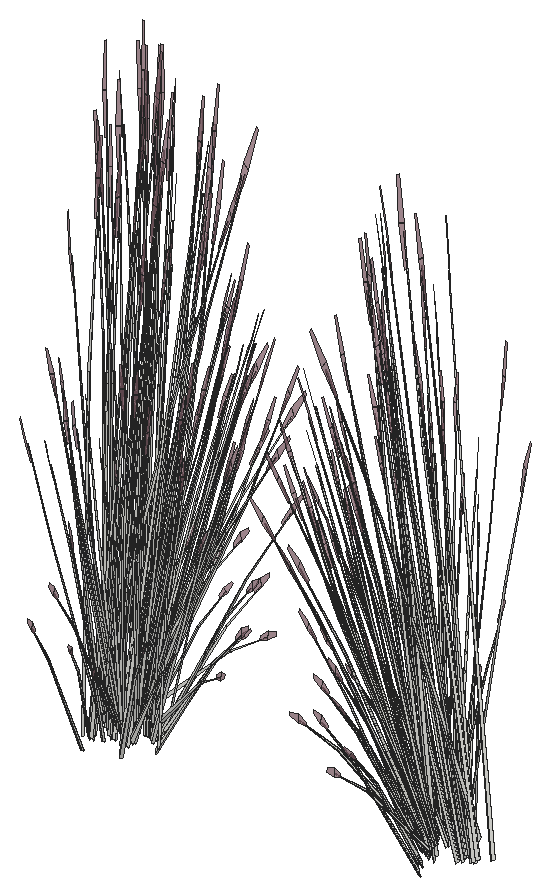
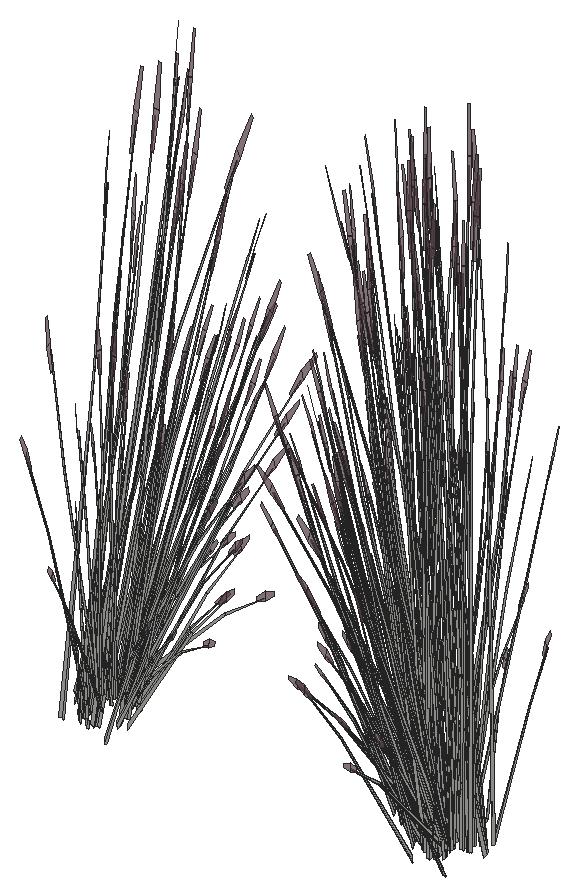
# SketchUp Ruby script. Lengths in inches.
U = 1.inch
M = Sketchup.active_model
def pt(a) = Geom::Point3d.new(a.map { |v| v * U })
def face(e, loops, mat)
  f = e.add_face(loops[0].map { |a| pt(a) })
  loops[1..].each { |l| e.add_face(l.map { |a| pt(a) }).erase! }
  f.material = f.back_material = mat if mat
  f
end
# faces: each face lists its corners as indices into pts; further lists are holes
def faces(e, pts, list, mat = nil) = list.each { |f| face(e, (f[0].is_a?(Array) ? f : [f]).map { |l| l.map { |i| pts[i] } }, mat) }
# xy, xz, yz: faces in a plane at the given z, y or x. An outline is a flat list of corners, or four numbers for a rectangle; further outlines are holes
def ring(l) = l.size == 4 ? [[l[0], l[1]], [l[2], l[1]], [l[2], l[3]], [l[0], l[3]]] : l.each_slice(2).to_a
def flat(e, list, mat, &to3) = list.each { |f| face(e, (f[0].is_a?(Array) ? f : [f]).map { |l| ring(l).map { |u, v| to3.(u, v) } }, mat) }
def xy(e, z, list, mat = nil) = flat(e, list, mat) { |x, y| [x, y, z] }
def xz(e, y, list, mat = nil) = flat(e, list, mat) { |x, z| [x, y, z] }
def yz(e, x, list, mat = nil) = flat(e, list, mat) { |y, z| [x, y, z] }
def lines(e, pts, list) = list.each { |a, b| e.add_line(pt(pts[a]), pt(pts[b])) }
# prism: a flat outline (further loops are holes) pulled along v
def prism(e, loops, v, mat = nil)
  f = face(e, loops, mat); d = Geom::Vector3d.new(v.map { |x| x * U })
  f.pushpull(f.normal.samedirection?(d) ? d.length : -d.length)
end
def box(e, o, s, mat = nil) = prism(e, [[o, [o[0] + s[0], o[1], o[2]], [o[0] + s[0], o[1] + s[1], o[2]], [o[0], o[1] + s[1], o[2]]]], [0, 0, s[2]], mat)
def at(x, y, z, deg = 0) = Geom::Transformation.translation(pt([x, y, z])) * Geom::Transformation.rotation(ORIGIN, Z_AXIS, deg.degrees)
def axes(o, x, y, z) = Geom::Transformation.new([*x, 0, *y, 0, *z, 0, *pt(o).to_a, 1])
def part(name) = M.definitions.add(name)
# library, detail: a bought-in or finely detailed component or shape, given as its bounding box
def library(name, o, s) = part(name).tap { |d| box(d.entities, o, s) }
def detail(e, o, s) = box(e.add_group.entities, o, s)
def put(e, d, t, mat = nil) = e.add_instance(d, t).tap { |i| i.material = mat if mat }
def group(e, t, mat = nil) = e.add_group.tap { |g| g.transformation = t; g.material = mat if mat }.entities
root = M.entities
M.materials.add("LightPink_Translucent").color = [144, 107, 117]
M.materials["LightPink_Translucent"].alpha = 0.75
c1 = part("blade")
p = [[2.15,0.21,22],[0,0.17,0],[0.09,0.45,0],[2.18,0.31,22],[2.29,0.31,22],[0.38,0.45,0],
  [2.48,0.24,33],[2.49,0.24,33],[2.48,0.22,33]]
faces(c1.entities,p,[[0,1,2,3],[4,5,2,3],[6,3,4,7],[8,0,3,6]])
c2 = part("seeds")
p = [[0.3,-0.1,1.38],[-0.01,-0.03,1.59],[-0.01,-0.03,0.03],[0.14,-0.07,-0.07],[0.29,-0.03,3],[0.15,0.01,3.11]]
faces(c2.entities,p,[[0,1,2,3],[1,0,4,5]],"LightPink_Translucent")
c3 = part("blade with seeds")
put(c3.entities,c1,at(0,0,0))
put(c3.entities,c2,axes([2.4,0.25,30.99],[1.5799,-0.05474,1.17369],[-0.12525,1.92788,0.29478],[-0.07173,-0.02425,1.56792]))
put(root,c3,axes([149.6,15.09,-3.67],[0.95122,0.19861,0.30756],[-0.23797,0.7099,-0.36492],[-0.15744,0.08885,1.64885]))
put(root,c3,axes([148.22,9.64,-4.51],[-0.12744,0.02202,1.76342],[-0.70477,-0.24781,-0.26939],[0.01183,-0.2067,0.30037]))
put(root,c3,axes([150.01,15.05,-3.52],[0.7111,-0.30552,0.49651],[0.42504,0.54784,0],[-0.16196,0.06958,1.57504]))
put(root,c3,axes([148.91,10.32,-1.47],[0.22906,-0.4699,-0.35414],[0.66828,0.13705,0.4572],[-0.06128,-0.18919,0.87481]))
put(root,c3,axes([147.79,12.86,-3.64],[0.33034,0.68327,0.45755],[-0.94388,0.2376,0.17955],[0.01154,-0.12555,1.58856]))
put(root,c3,axes([147.64,12.77,-3.79],[0.36864,-0.55059,-0.44739],[0.76598,0.26498,0.21531],[0,-0.12692,1.43643]))
put(root,c3,axes([148.58,14.55,-3.8],[-0.24791,-0.5268,0],[0.70791,-0.18448,0],[0,0,1.54371]))
put(root,c3,axes([147.68,15.66,-4.51],[0.12297,-0.03325,1.76342],[0.73967,0.18301,-0.26939],[0.02163,0.20626,0.30037]))
put(root,c3,axes([147.85,15.84,-1.47],[-0.22906,0.4699,-0.35414],[-0.66828,-0.13705,0.4572],[0.06128,0.18919,0.87481]))
put(root,c3,axes([149.58,13.51,-3.79],[-0.36864,0.55059,-0.44739],[-0.76598,-0.26498,0.21531],[0,0.12692,1.43643]))
put(root,c3,axes([149.19,10.39,-1.27],[0.55987,-0.20767,0.0643],[0.27403,0.37869,0.50621],[-0.05407,-0.16693,0.77189]))
put(root,c3,axes([147.37,16.68,-1.28],[0.09631,0.0984,1.74944],[0.77725,0.03866,-0.27667],[0.07816,0.217,0.14031]))
put(root,c3,axes([151.04,13.17,-3.53],[-0.59697,-0.44509,0.17642],[0.60159,-0.4317,0.35086],[-0.06593,0.0909,1.60407]))
put(root,c3,axes([148.98,12.92,-3.79],[0,-0.70701,0],[0.95008,0,0],[0,0,1.79456]))
put(root,c3,axes([148.99,10.43,-1.27],[0.74868,0.15974,0.48003],[-0.25601,0.52518,0.3958],[-0.04499,-0.20653,0.9933]))
put(root,c3,axes([148.1,13.04,-3.57],[0.8561,0.29616,0.24065],[-0.41201,0.61537,0.50002],[0,-0.14185,1.60543]))
put(root,c3,axes([149.46,13.2,-3.71],[0,0.70667,-0.05637],[-0.95008,0,0],[0,0.02221,1.79368]))
put(root,c3,axes([147.82,12.63,-3.28],[-0.82508,0.03772,0.44739],[-0.07462,-0.62614,-0.21531],[0.14771,-0.06346,1.43643]))
put(root,c3,axes([147.77,15.35,-0.95],[0.22906,-0.4699,0.35414],[0.66828,0.13705,-0.4572],[0.06128,0.18919,0.87481]))
put(root,c3,axes([147.43,11.56,-3.53],[-0.21949,0.60727,0.17642],[-0.8032,-0.17185,0.35086],[0.13875,-0.00296,1.60407]))
put(root,c3,axes([149,14.57,-3.71],[0.33034,0.70197,-0.06012],[-0.94388,0.24598,0],[0.01154,0.02451,1.72173]))
put(root,c3,axes([147.04,10.81,-3.625],[-0.47504,-0.61229,0],[0.79476,-0.34146,-0.51607],[0.18101,-0.07777,1.63711]))
put(root,c3,axes([147.91,15.42,-1.02],[0.36264,0.49684,-0.71045],[-0.74649,0.27689,0.08574],[0.0848,0.24006,1.00501]))
put(root,c3,axes([151.73,13.64,-3.8],[-0.94962,-0.00489,-0.04976],[0,-0.68292,0.49943],[-0.02984,0.15546,1.58352]))
put(root,c3,axes([149.86,11.59,-3.53],[-0.81646,0.16218,0.17642],[-0.20161,-0.60355,0.35086],[0.07282,0.08794,1.60407]))
put(root,c3,axes([149.03,9.33,-3.23],[0.09747,0.35631,1.1486],[-0.54071,-0.19735,0.84392],[0.05818,-0.18244,0.25299]))
put(root,c3,axes([148.67,17.03,-0.35],[0.52505,-0.35054,-0.06488],[0.48109,0.38392,-0.29416],[0.03387,0.10878,0.97024]))
put(root,c3,axes([148.53,12.47,-3.64],[-0.62999,0.55453,0.45755],[-0.74845,-0.4895,0.17955],[0.15188,-0.05534,1.58856]))
put(root,c3,axes([149.6,13.34,-3.79],[0.53038,0.39469,0],[-0.53038,0.39469,0],[0,0,1.69266]))
put(root,c3,axes([149.6,12.88,-3.28],[0.36864,-0.55059,0.44739],[0.76598,0.26498,-0.21531],[0,0.12692,1.43643]))
put(root,c3,axes([149.28,14.8,-3.8],[0.76598,0.27433,0],[-0.36864,0.57001,0],[0,0,1.74954]))
put(root,c3,axes([148.1875,15.52,-1.32],[0.7469,0.15318,-0.51099],[-0.25601,0.52518,-0.3958],[0.06849,0.21144,0.97773]))
put(root,c3,axes([147.55,15.55,-0.97],[0.74352,-0.28449,-0.1216],[0.36538,0.50492,-0.67495],[0.0981,0.21277,1.02557]))
put(root,c3,axes([149.35,12.75,-3.62],[-0.96033,-0.12874,0.49198],[0.19544,-0.7271,0.19306],[0.14034,0.07021,1.70813]))
put(root,c3,axes([151.35,9.91,-1.29],[-0.07716,0.04667,1.77383],[-0.75601,-0.15746,-0.16761],[-0.02737,-0.20368,0.31391]))
put(root,c3,axes([150.75,11.26,-0.97],[-0.83505,-0.03027,-0.1216],[0.02282,-0.57322,-0.67495],[0.05801,-0.22077,1.02557]))
put(root,c3,axes([151.53,13.74,-3.97],[-0.53038,0.38124,-0.30978],[-0.53038,-0.38124,0.30978],[0,0.1228,1.38974]))
put(root,c3,axes([150.02,13.67,-3.91],[0.2786,0.55945,-0.69212],[-0.80253,0.20149,-0.18165],[0.03079,0.18945,1.52773]))
put(root,c3,axes([149.625,13.07,-3.79],[0.85008,0,0],[0,0.63259,0],[0,0,1.78407]))
put(root,c3,axes([150.43,11.35,-0.95],[-0.5141,0.32171,0.35414],[-0.48666,-0.36734,-0.4572],[0.07405,-0.18664,0.87481]))
put(root,c3,axes([148.81,12.375,-3.28],[-0.45644,-0.51287,0.44739],[0.69137,-0.36116,-0.21531],[0.14771,0.06346,1.43643]))
put(root,c3,axes([147.98,12.5,-3.33],[-0.08854,-0.69723,-0.29095],[0.92215,-0.04216,-0.50002],[0.16238,-0.09287,1.59708]))
put(root,c3,axes([149.92,13.01,-3.38],[0.70791,-0.1782,0.1448],[0.24791,0.50885,-0.41347],[0,0.11199,1.26744]))
put(root,c3,axes([150.18,11.04,-1.32],[-0.54391,-0.41056,-0.51099],[0.57458,-0.35956,-0.3958],[0.08276,-0.2086,0.97773]))
put(root,c3,axes([149.68,13.05,-3.33],[0.85568,0.29155,-0.29095],[-0.41201,0.61537,-0.50002],[0.02689,0.15109,1.59708]))
put(root,c3,axes([147.85,10.95,-3.97],[0.70886,0.15119,-0.30978],[-0.17848,0.53243,0.30978],[0.1429,-0.0614,1.38974]))
put(root,c3,axes([149.83,10.3125,-3.41],[-0.21597,0.12368,1.43002],[-0.64681,-0.21647,-0.30754],[0.1199,-0.26922,0.61141]))
put(root,c3,axes([151.53,13.19,-3.52],[0,-0.61104,0.49651],[0.85008,0,0],[0,0.13917,1.57504]))
put(root,c3,axes([151.9,13.76,-3.98],[0,0.61104,-0.49651],[-0.85008,0,0],[0,0.13917,1.57504]))
put(root,c3,axes([149.63,15.61,-1.27],[-0.75571,0.14023,0.48003],[-0.13115,-0.55007,0.3958],[0.17773,0.16212,0.9933]))
put(root,c3,axes([147.6875,10.71,-3.98],[0.7111,-0.30552,-0.49651],[0.42504,0.54784,0],[0.16196,-0.06958,1.57504]))
put(root,c3,axes([149.48,15.72,-1.27],[-0.34533,0.38816,0.0643],[-0.49176,-0.22599,0.50621],[0.15898,0.12445,0.77189]))
put(root,c3,axes([148.61,14.4375,-2.125],[-0.17368,-0.19618,1.71376],[0.80256,-0.16516,0.13857],[0.18139,0.30799,0.73262]))
put(root,c3,axes([149.11,12.23,-3.38],[0.14658,-0.54532,0.1448],[0.71613,0.09466,-0.41347],[0.13033,0.05599,1.26744]))
put(root,c3,axes([150.13,11.28,-3.52],[-0.7111,-0.30552,0.49651],[0.42504,-0.54784,0],[0.16196,0.06958,1.57504]))
put(root,c3,axes([150.35,11.23,-1.02],[0.01977,-0.56521,-0.71045],[0.83252,0.03796,0.08574],[0.08786,-0.23945,1.00501]))
put(root,c3,axes([149.51,14.47,-3.82],[0.79769,-0.20732,-0.19198],[0.2803,0.59721,0.00008],[0.08805,-0.02292,1.73897]))
put(root,c3,axes([149.375,15.27,-0.95],[-0.11735,-0.49217,0.35414],[0.67083,-0.12996,-0.4572],[0.18018,0.14104,0.87481]))
put(root,c3,axes([149.53,12.7,-3.79],[0.45644,0.51287,-0.44739],[-0.69137,0.36116,0.21531],[0.14771,0.06346,1.43643]))
put(root,c3,axes([149.83,12.44,-1.53],[-0.65655,-0.31748,1.38283],[0.69326,-0.49431,0.59665],[0.21183,0.29789,1.33663]))
put(root,c3,axes([150.69,10.89,-1.47],[0.5141,-0.32171,-0.35414],[0.48666,0.36734,0.4572],[0.07405,-0.18664,0.87481]))
put(root,c3,axes([148.72,15.96,-1.29],[0.00225,-0.07398,1.77383],[0.65113,-0.32638,-0.16761],[0.22617,0.1165,0.31391]))
put(root,c3,axes([150.89,11.05,-1.27],[0.62439,0.02847,0.0643],[-0.01712,0.42991,0.50621],[0.06534,-0.16468,0.77189]))
put(root,c3,axes([150.82,15.02,-3.23],[-0.4278,-0.1757,1.1486],[0.5524,-0.17852,0.84392],[0.14899,0.15122,0.25299]))
put(root,c3,axes([149.29,14.84,-3.41],[0.01341,-0.20255,1.43002],[0.64074,-0.22625,-0.30754],[0.1978,0.24243,0.61141]))
put(root,c3,axes([151.51,10.35,-1.28],[-0.00733,-0.12161,1.74944],[-0.61946,-0.35147,-0.27667],[0.09577,-0.21306,0.14031]))
put(root,c3,axes([148.53,11.97,-3.94],[0.51177,-0.45928,-0.62353],[0.63575,0.41646,-0.16365],[0.20507,-0.11457,1.37633]))
put(root,c3,axes([150.69,11.01,-1.27],[0.54105,0.41691,0.48003],[-0.57458,0.35956,0.3958],[0.0998,-0.1956,0.9933]))
put(root,c3,axes([150.78,11.56,-3.97],[0.17848,0.53243,-0.30978],[-0.70886,0.15119,0.30978],[0.1429,0.0614,1.38974]))
put(root,c3,axes([152.11,13.29,-3.625],[0.95008,0,0],[0,0.68292,-0.51607],[0,0.15554,1.63711]))
put(root,c3,axes([149.04,12.41,-3.33],[0.76714,-0.40567,-0.29095],[0.51013,0.57321,-0.50002],[0.18927,0.05821,1.59708]))
put(root,c3,axes([150.89,15.82,-3.33],[-0.48723,-0.01916,1.0506],[0.32177,-0.40701,0.58006],[0.19248,0.1446,0.8241]))
put(root,c3,axes([151.32,12.34,-0.95],[-0.66138,0.08733,0.35414],[-0.17464,-0.49921,-0.4572],[0.18953,-0.13408,0.87481]))
put(root,c3,axes([149.41,10.94,-2.125],[-0.14147,0.21002,1.71376],[-0.59349,-0.43464,0.13857],[0.26773,-0.27089,0.73262]))
put(root,c3,axes([149.31,15.53,-0.97],[0.45276,-0.52302,-0.1216],[0.65568,0.30132,-0.67495],[0.22792,0.14777,1.02557]))
put(root,c3,axes([147.1,12.05,-4.41],[-0.74787,0.24464,1.28929],[-0.23804,-0.70192,0.50096],[0.45924,0.01168,1.46642]))
put(root,c3,axes([151.66,12.39,-0.97],[-0.70283,-0.33692,-0.1216],[0.40491,-0.48793,-0.67495],[0.19857,-0.16961,1.02557]))
put(root,c3,axes([149.85,15.27,-1.32],[0.74975,-0.14525,-0.51099],[0.13115,0.55007,-0.3958],[0.20138,0.15763,0.97773]))
put(root,c3,axes([150.54,10.96,-3.625],[0.47504,-0.61229,0],[0.79476,0.34146,-0.51607],[0.18101,0.07777,1.63711]))
put(root,c3,axes([151.34,10.69,-4.51],[-0.11372,-0.04814,1.76342],[-0.29211,-0.53779,-0.26939],[0.19706,-0.14594,0.30037]))
put(root,c3,axes([150.71,14.61,-0.95],[-0.43232,-0.38257,0.35414],[0.49364,-0.36215,-0.4572],[0.25081,0.0551,0.87481]))
put(root,c3,axes([150.97,11.33,-3.98],[0.7111,0.30552,-0.49651],[-0.42504,0.54784,0],[0.16196,0.06958,1.57504]))
put(root,c3,axes([151.1,14.95,-1.27],[-0.03826,0.46465,0.0643],[-0.57772,-0.01274,0.50621],[0.2213,0.04862,0.77189]))
put(root,c3,axes([150.9375,15.68,-4.51],[0.05536,-0.08822,1.76342],[0.69692,-0.25981,-0.26939],[0.21129,0.13447,0.30037]))
put(root,c3,axes([151.16,14.81,-1.27],[-0.56024,0.40262,0.48003],[-0.48318,-0.42758,0.3958],[0.26285,0.07427,0.9933]))
put(root,c3,axes([151.3125,11.99,-1.32],[-0.19519,-0.55794,-0.51099],[0.73919,-0.0976,-0.3958],[0.21183,-0.14986,0.97773]))
put(root,c3,axes([152.61,14.87,-2.07],[-0.14542,-0.51365,-0.03492],[0.68734,-0.11809,-0.15832],[0.14353,0.03256,0.52218]))
put(root,c3,axes([151.42,13.53,-0.95],[-0.63144,-0.17046,0.35414],[0.18417,-0.49731,-0.4572],[0.25423,-0.0456,0.87481]))
put(root,c3,axes([149.9375,12.5,-3.94],[0.79037,0.10018,-0.62353],[-0.16679,0.61794,-0.16365],[0.23587,0.07488,1.37633]))
put(root,c3,axes([153.3,12.86,-3.74],[-0.47106,-0.39072,-0.06488],[0.51591,-0.35801,-0.29416],[0.14618,-0.02521,0.97024]))
put(root,c3,axes([152.22,10.875,-3.23],[-0.25308,0.31105,1.1486],[-0.21753,-0.4179,0.84392],[0.20902,-0.10472,0.25299]))
put(root,c3,axes([151.92,12.26,-1.27],[0.52161,0.25698,0.0643],[-0.30368,0.36595,0.50621],[0.16723,-0.11831,0.77189]))
put(root,c3,axes([151.77,12.15,-1.27],[0.18844,0.56237,0.48003],[-0.73919,0.0976,0.3958],[0.21785,-0.13226,0.9933]))
put(root,c3,axes([149.77,13.83,-2.125],[-0.28223,-0.10528,1.71376],[0.58406,-0.44165,0.13857],[0.36402,0.19924,0.73262]))
put(root,c3,axes([153.39,12.24,-1.29],[-0.09924,-0.00464,1.77383],[-0.4121,-0.49725,-0.16761],[0.1655,-0.1635,0.31391]))
put(root,c3,axes([151.86,12.04,-1.47],[0.66138,-0.08733,-0.35414],[0.17464,0.49921,0.4572],[0.18953,-0.13408,0.87481]))
put(root,c3,axes([151.33,12.21,-1.02],[0.39688,-0.48213,-0.71045],[0.69548,0.34264,0.08574],[0.23697,-0.17468,1.00501]))
put(root,c3,axes([152,13.6875,-1.27],[0.27906,0.41663,0.0643],[-0.50888,0.20393,0.50621],[0.22432,-0.04024,0.77189]))
put(root,c3,axes([151.33,14.81,-1.47],[0.43232,0.38257,-0.35414],[-0.49364,0.36215,0.4572],[0.25081,0.0551,0.87481]))
put(root,c3,axes([150.83,14.85,-0.97],[0.04068,-0.62141,-0.1216],[0.77029,0.01698,-0.67495],[0.29667,0.04317,1.02557]))
put(root,c3,axes([151.69,13.7,-0.97],[-0.38229,-0.5533,-0.1216],[0.6785,-0.2719,-0.67495],[0.28593,-0.073,1.02557]))
put(root,c3,axes([151.94,13.54,-1.27],[-0.21466,0.55714,0.48003],[-0.70573,-0.19051,0.3958],[0.27753,-0.03348,0.9933]))
put(root,c3,axes([151.5,14.48,-1.28],[0.16299,-0.01033,1.74944],[0.44707,-0.47471,-0.27667],[0.28992,0.06266,0.14031]))
put(root,c3,axes([151.66,13.22,-1.32],[0.20584,-0.55581,-0.51099],[0.70573,0.19051,-0.3958],[0.28414,-0.05097,0.97773]))
put(root,c3,axes([153.43,13.58,-3.23],[-0.46945,0.10088,1.1486],[0.22097,-0.4169,0.84392],[0.24904,0.02853,0.25299]))
put(root,c3,axes([151.91,11.77,-3.41],[-0.27143,-0.0181,1.43002],[-0.27808,-0.48551,-0.30754],[0.33346,-0.13735,0.61141]))
put(root,c3,axes([152.09,13.48,-1.47],[0.63144,0.17046,-0.35414],[-0.18417,0.49731,0.4572],[0.25423,-0.0456,0.87481]))
put(root,c3,axes([150.87,14.55,-1.02],[0.75952,0.01471,-0.71045],[-0.05101,0.61953,0.08574],[0.32177,0.06538,1.00501]))
put(root,c3,axes([152.41,13.38,-4.02],[-0.48937,0.07333,1.41583],[-0.07789,-0.58369,0.08104],[0.34275,-0.08835,0.80566]))
put(root,c3,axes([152.94,13,-4.51],[-0.03971,-0.09277,1.76342],[0.27541,-0.54264,-0.26939],[0.27782,-0.00781,0.30037]))
put(root,c3,axes([153.21,15.34,-1.29],[-0.0687,-0.05349,1.77383],[0.15029,-0.57341,-0.16761],[0.27062,-0.03664,0.31391]))
put(root,c3,axes([150.37,12.86,-2.125],[-0.31515,0.01384,1.71376],[0.20907,-0.5998,0.13857],[0.44912,0.0371,0.73262]))
put(root,c3,axes([151.52,13.43,-1.02],[0.66765,-0.26986,-0.71045],[0.37208,0.55551,0.08574],[0.32259,-0.0631,1.00501]))
put(root,c3,axes([153.77,12.83,-1.28],[0.10543,-0.09307,1.74944],[-0.13495,-0.57092,-0.27667],[0.26455,-0.10825,0.14031]))
put(root,c3,axes([152.55,14.25,-3.41],[-0.18299,-0.15028,1.43002],[0.23809,-0.49714,-0.30754],[0.37023,0.06735,0.61141]))
put(root,c3,axes([181.36,12.17,-2.125],[0.31515,-0.01384,1.71376],[-0.20907,0.5998,0.13857],[-0.44912,-0.0371,0.73262]))
put(root,c3,axes([181.49,13.23,-2.125],[0.26363,-0.12925,1.71376],[0.22195,0.59723,0.13857],[-0.41388,0.13498,0.73262]))
put(root,c3,axes([180.67,14.24,-3.41],[0.26405,0.05016,1.43002],[0.17019,0.51235,-0.30754],[-0.35868,0.0959,0.61141]))
put(root,c3,axes([183.01,12.6,-2.66],[0.21597,-0.08839,1.77064],[0.07448,0.61717,0.13857],[-0.4678,0.08189,0.63284]))
put(root,c3,axes([180.6875,13.02,-1.28],[-0.12407,0.07933,1.74944],[0.01055,0.57963,-0.27667],[-0.2844,0.07538,0.14031]))
put(root,c3,axes([182.31,11.61,-1.02],[-0.75952,-0.01471,-0.71045],[0.05101,-0.61953,0.08574],[-0.32177,-0.06538,1.00501]))
put(root,c3,axes([181.69,11.76,-3.41],[0.14835,0.17012,1.43002],[-0.34183,0.46242,-0.30754],[-0.351,-0.11053,0.61141]))
put(root,c3,axes([181.09,12.6875,-1.47],[-0.63144,-0.17046,-0.35414],[0.18417,-0.49731,0.4572],[-0.25423,0.0456,0.87481]))
put(root,c3,axes([181.96,11.21,-2.125],[0.28223,0.10528,1.71376],[-0.58406,0.44165,0.13857],[-0.36402,-0.19924,0.73262]))
put(root,c3,axes([179.31,13.6,-1.29],[0.09697,0.01639,1.77383],[0.29997,0.53988,-0.16761],[-0.1985,0.1417,0.31391]))
put(root,c3,axes([181.52,12.94,-1.32],[-0.20584,0.55581,-0.51099],[-0.70573,-0.19051,-0.3958],[-0.28414,0.05097,0.97773]))
put(root,c3,axes([182.05,11.74,-1.32],[-0.55171,0.40476,-0.51099],[-0.48318,-0.42758,-0.3958],[-0.28031,-0.06159,0.97773]))
put(root,c3,axes([181.16,12.91,-4.51],[0.01927,0.0963,1.76342],[-0.38846,0.5029,-0.26939],[-0.27592,-0.02535,0.30037]))
put(root,c3,axes([181.27,10.6,-1.29],[0.05633,0.06098,1.77383],[-0.27155,0.54815,-0.16761],[-0.27501,0.00397,0.31391]))
put(root,c3,axes([180.12,15.32,-3.23],[0.31665,-0.27694,1.1486],[0.12495,0.43841,0.84392],[-0.22883,0.0785,0.25299]))
put(root,c3,axes([181.9,10.24,-1.28],[-0.16348,-0.00431,1.74944],[-0.52047,0.43131,-0.27667],[-0.2777,-0.08813,0.14031]))
put(root,c3,axes([181.23,12.625,-1.27],[0.21466,-0.55714,0.48003],[0.70573,0.19051,0.3958],[-0.27753,0.03348,0.9933]))
put(root,c3,axes([181.48,12.46,-0.97],[0.38229,0.5533,-0.1216],[-0.6785,0.2719,-0.67495],[-0.28593,0.073,1.02557]))
put(root,c3,axes([182.34,11.32,-0.97],[-0.04068,0.62141,-0.1216],[-0.77029,-0.01698,-0.67495],[-0.29667,-0.04317,1.02557]))
put(root,c3,axes([181.85,11.36,-1.47],[-0.43232,-0.38257,-0.35414],[0.49364,-0.36215,0.4572],[-0.25081,-0.0551,0.87481]))
put(root,c3,axes([181.18,12.48,-1.27],[-0.27906,-0.41663,0.0643],[0.50888,-0.20393,0.50621],[-0.22432,0.04024,0.77189]))
put(root,c3,axes([182.46,13.63,-2.125],[0.18977,-0.18775,1.71376],[0.47917,0.50677,0.13857],[-0.32866,0.23079,0.73262]))
put(root,c3,axes([181.32,14.12,-1.47],[-0.66138,0.08733,-0.35414],[-0.17464,-0.49921,0.4572],[-0.18953,0.13408,0.87481]))
put(root,c3,axes([180.96,15.6,-4.51],[0.10192,0.06105,1.76342],[0.17281,0.56562,-0.26939],[-0.22588,0.12062,0.30037]))
put(root,c3,axes([180.81,12.28,-3.23],[0.48508,-0.04372,1.1486],[-0.3077,0.38525,0.84392],[-0.23971,-0.05779,0.25299]))
put(root,c3,axes([181.4,14.01,-1.27],[-0.18844,-0.56237,0.48003],[0.73919,-0.0976,0.3958],[-0.21785,0.13226,0.9933]))
put(root,c3,axes([181.78,11.21,-0.91],[0.62747,-0.45094,0.53763],[0.54116,0.47889,0.4433],[-0.29439,-0.08318,1.11249]))
put(root,c3,axes([181.26,13.9,-1.27],[-0.52161,-0.25698,0.0643],[0.30368,-0.36595,0.50621],[-0.16723,0.11831,0.77189]))
put(root,c3,axes([182.32,14.09,-2.125],[0.14147,-0.21002,1.71376],[0.59349,0.43464,0.13857],[-0.26773,0.27089,0.73262]))
put(root,c3,axes([181.75,12.63,-0.95],[0.63144,0.17046,0.35414],[-0.18417,0.49731,-0.4572],[-0.25423,0.0456,0.87481]))
put(root,c3,axes([181.86,14.18,-1.32],[0.19519,0.55794,-0.51099],[-0.73919,0.0976,-0.3958],[-0.21183,0.14986,0.97773]))
put(root,c3,axes([182.07,11.21,-1.27],[0.03826,-0.46465,0.0643],[0.57772,0.01274,0.50621],[-0.2213,-0.04862,0.77189]))
put(root,c3,axes([180.71,15.18,-1.28],[-0.01889,0.12092,1.74944],[0.53598,0.42065,-0.27667],[-0.14032,0.19892,0.14031]))
put(root,c3,axes([183.7,13.78,-3.94],[-0.79037,-0.10018,-0.62353],[0.16679,-0.61794,-0.16365],[-0.23587,-0.07488,1.37633]))
put(root,c3,axes([183.85,10.41,-0.57],[-0.50709,0.58578,-0.13619],[-0.73436,-0.33748,-0.75594],[-0.25527,-0.1655,1.14864]))
put(root,c3,axes([182.46,11.56,-0.95],[0.43232,0.38257,0.35414],[-0.49364,0.36215,-0.4572],[-0.25081,-0.0551,0.87481]))
put(root,c3,axes([183.625,10.88,-1.02],[-0.64788,-0.29534,-0.71045],[0.46044,-0.51755,0.08574],[-0.23473,-0.17635,1.00501]))
put(root,c3,axes([183.32,10.9,-1.32],[-0.74975,0.14525,-0.51099],[-0.13115,-0.55007,-0.3958],[-0.20138,-0.15763,0.97773]))
put(root,c3,axes([182.67,14.95,-3.98],[-0.7111,-0.30552,-0.49651],[0.42504,-0.54784,0],[-0.16196,-0.06958,1.57504]))
put(root,c3,axes([182.36,10.4,-4.51],[-0.0736,0.08049,1.76342],[-0.74378,0.17355,-0.26939],[-0.17968,-0.15788,0.30037]))
put(root,c3,axes([181.51,13.78,-0.97],[0.70283,0.33692,-0.1216],[-0.40491,0.48793,-0.67495],[-0.19857,0.16961,1.02557]))
put(root,c3,axes([183.1,15.32,-3.625],[-0.47504,0.61229,0],[-0.79476,-0.34146,-0.51607],[-0.18101,-0.07777,1.63711]))
put(root,c3,axes([180.35,15.24,-0.35],[0.67048,0.16311,-0.06488],[-0.20625,0.50201,-0.29416],[-0.10966,0.07622,0.97024]))
put(root,c3,axes([181.86,13.83,-0.95],[0.66138,-0.08733,0.35414],[0.17464,0.49921,-0.4572],[-0.18953,0.13408,0.87481]))
put(root,c3,axes([182.23,16.2,-3.41],[0.23977,-0.09639,1.43002],[0.59198,0.29065,-0.30754],[-0.1762,0.25149,0.61141]))
put(root,c3,axes([181.89,10.71,-3.87],[-0.21918,0.49894,-0.03893],[-0.6746,-0.15348,-0.17649],[-0.10242,-0.08161,0.58215]))
put(root,c3,axes([183.65,9.02,-1.29],[-0.01417,0.07324,1.77383],[-0.6991,0.2658,-0.16761],[-0.20573,-0.13587,0.31391]))
put(root,c3,axes([182.9,10.08,-3.41],[-0.04601,0.19989,1.43002],[-0.67263,0.16733,-0.30754],[-0.15723,-0.25836,0.61141]))
put(root,c3,axes([183.12,10.6,-2.125],[0.17368,0.19618,1.71376],[-0.80256,0.16516,0.13857],[-0.18139,-0.30799,0.73262]))
put(root,c3,axes([184.6,13.87,-3.33],[-0.76714,0.40567,-0.29095],[-0.51013,-0.57321,-0.50002],[-0.18927,-0.05821,1.59708]))
put(root,c3,axes([182.48,15.15,-1.27],[-0.54105,-0.41691,0.48003],[0.57458,-0.35956,0.3958],[-0.0998,0.1956,0.9933]))
put(root,c3,axes([183.4,10.49,-1.47],[-0.11735,-0.49217,-0.35414],[0.67083,-0.12996,0.4572],[-0.18018,-0.14104,0.87481]))
put(root,c3,axes([181.53,12.99,-3.625],[-0.95008,0,0],[0,-0.68292,-0.51607],[0,-0.15554,1.63711]))
put(root,c3,axes([182.87,14.72,-3.97],[-0.17848,-0.53243,-0.30978],[0.70886,-0.15119,0.30978],[-0.1429,-0.0614,1.38974]))
put(root,c3,axes([182.28,15.11,-1.27],[-0.62439,-0.02847,0.0643],[0.01712,-0.42991,0.50621],[-0.06534,0.16468,0.77189]))
put(root,c3,axes([182.48,15.28,-1.47],[-0.5141,0.32171,-0.35414],[-0.48666,-0.36734,0.4572],[-0.07405,0.18664,0.87481]))
put(root,c3,axes([185.11,14.3125,-3.94],[-0.51177,0.45928,-0.62353],[-0.63575,-0.41646,-0.16365],[-0.20507,0.11457,1.37633]))
put(root,c3,axes([183.8,10.89,-0.95],[0.11735,0.49217,0.35414],[-0.67083,0.12996,-0.4572],[-0.18018,-0.14104,0.87481]))
put(root,c3,axes([180.65,16.42,-1.29],[0.0862,-0.03689,1.77383],[0.71245,0.24539,-0.16761],[-0.01674,0.20431,0.31391]))
put(root,c3,axes([182.27,12.81,-3.67],[-0.70674,0.51372,0.30756],[-0.70717,-0.50832,-0.36492],[-0.02468,-0.14589,1.64885]))
put(root,c3,axes([185.18,14.22,-2.67],[0.65659,0.2464,1.51261],[-0.64324,0.53082,0.59816],[-0.28812,-0.31461,1.26806]))
put(root,c3,axes([182.67,9.76,-3.23],[0.39634,0.21267,1.1486],[-0.57721,0.12784,0.84392],[-0.1235,-0.16344,0.25299]))
put(root,c3,axes([185.46,14.05,-3.54],[-0.74193,-0.49181,-0.25192],[0.6243,-0.55226,0.5513],[-0.19979,0.05753,1.68216]))
put(root,c3,axes([184.11,13.58,-3.79],[-0.45644,-0.51287,-0.44739],[0.69137,-0.36116,0.21531],[-0.14771,-0.06346,1.43643]))
put(root,c3,axes([182.82,14.9375,-0.66],[-0.01977,0.56521,-0.7886],[-0.83252,-0.03796,0.09517],[-0.08786,0.23945,1.11556]))
put(root,c3,axes([182.81,16.53,-3.23],[-0.01966,-0.36332,1.1486],[0.49135,0.25914,0.84392],[-0.09663,0.17317,0.25299]))
put(root,c3,axes([183.5,10.31,-0.91],[0.84639,-0.15705,0.53763],[0.14689,0.61608,0.4433],[-0.19906,-0.18157,1.11249]))
put(root,c3,axes([185.09,13.95,-3.79],[-0.82508,0.03772,-0.44739],[-0.07462,-0.62614,0.21531],[-0.14771,0.06346,1.43643]))
put(root,c3,axes([183.69,10.45,-1.27],[0.34533,-0.38816,0.0643],[0.49176,0.22599,0.50621],[-0.15898,-0.12445,0.77189]))
put(root,c3,axes([183.51,15,-3.52],[0.7111,0.30552,0.49651],[-0.42504,0.54784,0],[-0.16196,-0.06958,1.57504]))
put(root,c3,axes([182.54,15.73,-2.64],[0.01669,-0.31544,1.54345],[0.75083,0.16661,0.21329],[-0.06506,0.33618,0.72882]))
put(root,c3,axes([184.18,13.875,-3.5625],[0.20138,-0.72405,-0.23429],[0.95485,0.12621,0.51271],[-0.16685,-0.09999,1.5644]))
put(root,c3,axes([184.53,14.05,-3.38],[-0.14658,0.54532,0.1448],[-0.71613,-0.09466,-0.41347],[-0.13033,-0.05599,1.26744]))
put(root,c3,axes([184.45,9.3,-1.28],[-0.11621,-0.08567,1.74944],[-0.77555,0.05431,-0.27667],[-0.12378,-0.20491,0.14031]))
put(root,c3,axes([185.95,15.57,-3.98],[-0.7111,0.30552,-0.49651],[-0.42504,-0.54784,0],[-0.16196,0.06958,1.57504]))
put(root,c3,axes([181.74,12.52,-3.98],[0,-0.61104,-0.49651],[0.85008,0,0],[0,-0.13917,1.57504]))
